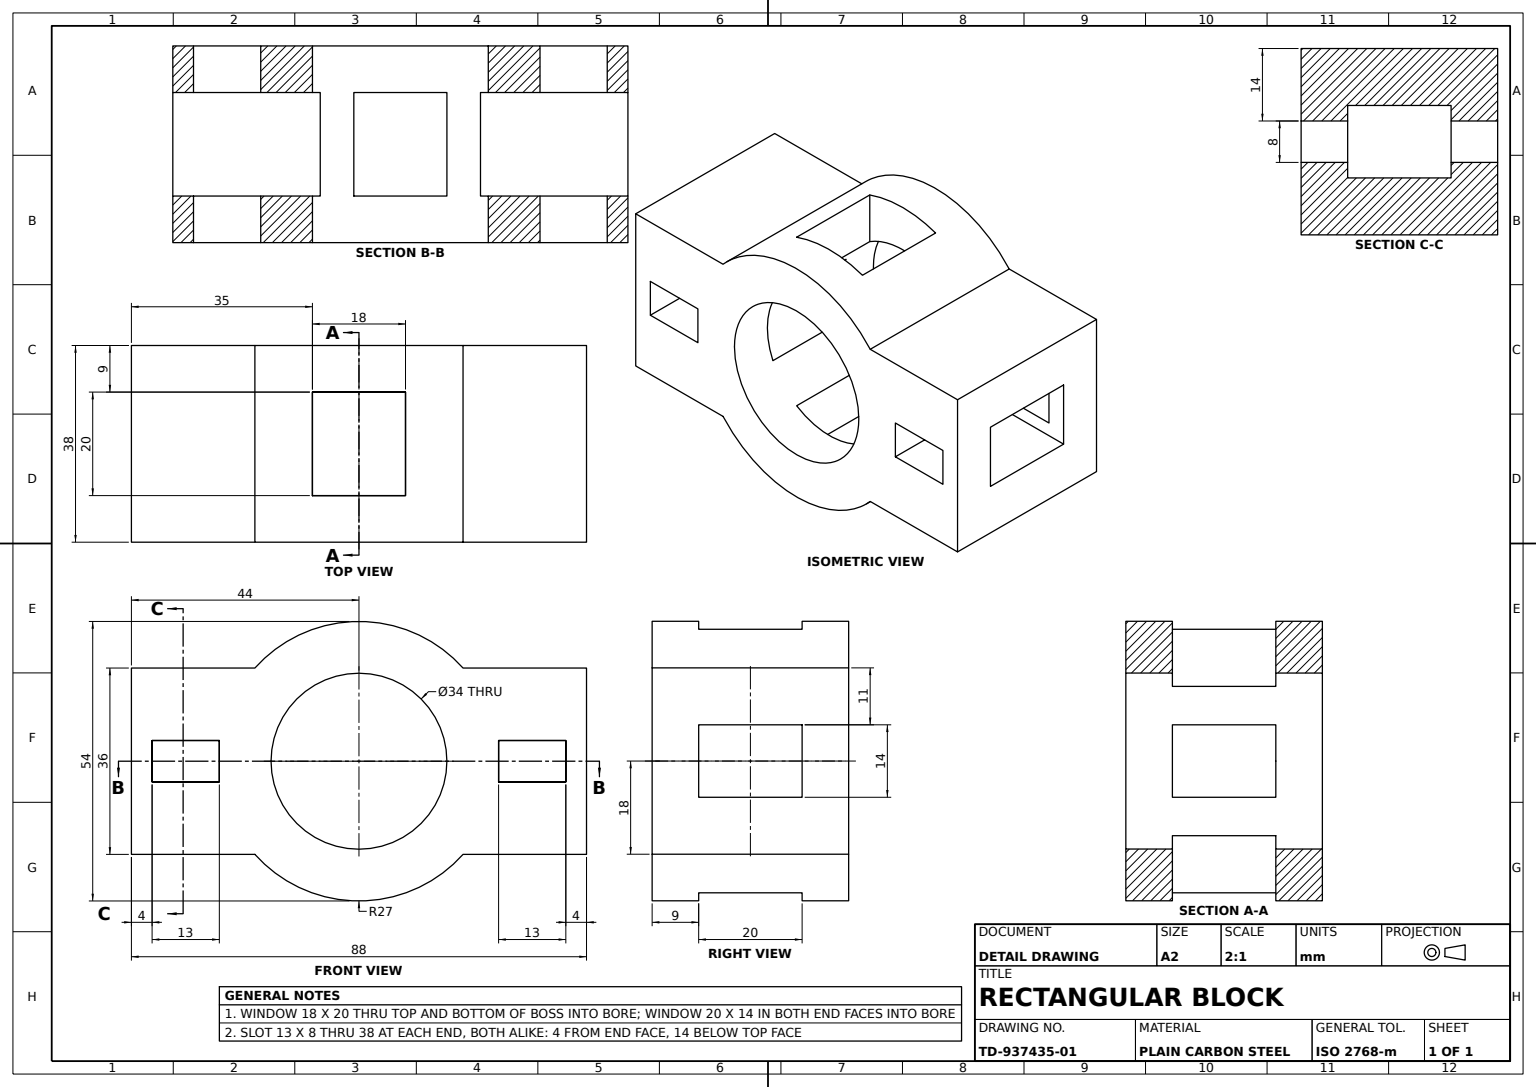
ISO-10303-21;
HEADER;
FILE_DESCRIPTION((''),'2;1');
FILE_NAME('','',(''),(''),'','','');
FILE_SCHEMA(('AUTOMOTIVE_DESIGN'));
ENDSEC;
DATA;
#1=APPLICATION_CONTEXT('');
#2=PRODUCT_CONTEXT('',#1,'mechanical');
#3=PRODUCT('','','',(#2));
#4=PRODUCT_DEFINITION_FORMATION('','',#3);
#5=PRODUCT_DEFINITION_CONTEXT('',#1,'design');
#6=PRODUCT_DEFINITION('','',#4,#5);
#7=PRODUCT_DEFINITION_SHAPE('','',#6);
#8=(LENGTH_UNIT()NAMED_UNIT(*)SI_UNIT(.MILLI.,.METRE.));
#9=(NAMED_UNIT(*)PLANE_ANGLE_UNIT()SI_UNIT($,.RADIAN.));
#10=(NAMED_UNIT(*)SI_UNIT($,.STERADIAN.)SOLID_ANGLE_UNIT());
#11=UNCERTAINTY_MEASURE_WITH_UNIT(LENGTH_MEASURE(1.E-05),#8,'distance_accuracy_value','');
#12=(GEOMETRIC_REPRESENTATION_CONTEXT(3)GLOBAL_UNCERTAINTY_ASSIGNED_CONTEXT((#11))GLOBAL_UNIT_ASSIGNED_CONTEXT((#8,#9,#10))REPRESENTATION_CONTEXT('',''));
#13=CARTESIAN_POINT('',(9.,14.422205,-29.));
#14=VERTEX_POINT('',#13);
#15=CARTESIAN_POINT('',(9.,14.422205,-9.));
#16=VERTEX_POINT('',#15);
#17=CARTESIAN_POINT('',(9.,14.422205,-38.));
#18=DIRECTION('',(0.,0.,1.));
#19=VECTOR('',#18,1000.);
#20=LINE('',#17,#19);
#21=EDGE_CURVE('',#14,#16,#20,.T.);
#22=ORIENTED_EDGE('',*,*,#21,.T.);
#23=CARTESIAN_POINT('',(9.,25.455844,-9.));
#24=VERTEX_POINT('',#23);
#25=CARTESIAN_POINT('',(9.,27.,-9.));
#26=DIRECTION('',(0.,-1.,0.));
#27=VECTOR('',#26,1000.);
#28=LINE('',#25,#27);
#29=EDGE_CURVE('',#24,#16,#28,.T.);
#30=ORIENTED_EDGE('',*,*,#29,.F.);
#31=CARTESIAN_POINT('',(9.,25.455844,-29.));
#32=VERTEX_POINT('',#31);
#33=CARTESIAN_POINT('',(9.,25.455844,-38.));
#34=LINE('',#33,#19);
#35=EDGE_CURVE('',#32,#24,#34,.T.);
#36=ORIENTED_EDGE('',*,*,#35,.F.);
#37=CARTESIAN_POINT('',(9.,27.,-29.));
#38=LINE('',#37,#27);
#39=EDGE_CURVE('',#32,#14,#38,.T.);
#40=ORIENTED_EDGE('',*,*,#39,.T.);
#41=EDGE_LOOP('',(#22,#30,#36,#40));
#42=FACE_OUTER_BOUND('',#41,.T.);
#43=DIRECTION('',(-1.,0.,0.));
#44=AXIS2_PLACEMENT_3D('',#25,#43,#18);
#45=PLANE('',#44);
#46=ADVANCED_FACE('',(#42),#45,.T.);
#47=CARTESIAN_POINT('',(44.,7.,-9.));
#48=VERTEX_POINT('',#47);
#49=CARTESIAN_POINT('',(15.491933,7.,-9.));
#50=VERTEX_POINT('',#49);
#51=VECTOR('',#43,1000.);
#52=LINE('',#47,#51);
#53=EDGE_CURVE('',#48,#50,#52,.T.);
#54=ORIENTED_EDGE('',*,*,#53,.F.);
#55=CARTESIAN_POINT('',(44.,-7.,-9.));
#56=VERTEX_POINT('',#55);
#57=DIRECTION('',(0.,1.,0.));
#58=VECTOR('',#57,1000.);
#59=LINE('',#55,#58);
#60=EDGE_CURVE('',#56,#48,#59,.T.);
#61=ORIENTED_EDGE('',*,*,#60,.F.);
#62=CARTESIAN_POINT('',(15.491933,-7.,-9.));
#63=VERTEX_POINT('',#62);
#64=LINE('',#55,#51);
#65=EDGE_CURVE('',#56,#63,#64,.T.);
#66=ORIENTED_EDGE('',*,*,#65,.T.);
#67=CARTESIAN_POINT('',(17.,0.,-9.));
#68=VERTEX_POINT('',#67);
#69=CARTESIAN_POINT('',(0.,0.,-9.));
#70=DIRECTION('',(0.,0.,-1.));
#71=DIRECTION('',(1.,0.,0.));
#72=AXIS2_PLACEMENT_3D('',#69,#70,#71);
#73=CIRCLE('',#72,17.);
#74=EDGE_CURVE('',#68,#63,#73,.T.);
#75=ORIENTED_EDGE('',*,*,#74,.F.);
#76=EDGE_CURVE('',#50,#68,#73,.T.);
#77=ORIENTED_EDGE('',*,*,#76,.F.);
#78=EDGE_LOOP('',(#54,#61,#66,#75,#77));
#79=FACE_OUTER_BOUND('',#78,.T.);
#80=CARTESIAN_POINT('',(27.,4.,-9.));
#81=VERTEX_POINT('',#80);
#82=CARTESIAN_POINT('',(40.,4.,-9.));
#83=VERTEX_POINT('',#82);
#84=VECTOR('',#71,1000.);
#85=LINE('',#82,#84);
#86=EDGE_CURVE('',#81,#83,#85,.T.);
#87=ORIENTED_EDGE('',*,*,#86,.F.);
#88=CARTESIAN_POINT('',(27.,-4.,-9.));
#89=VERTEX_POINT('',#88);
#90=LINE('',#88,#58);
#91=EDGE_CURVE('',#89,#81,#90,.T.);
#92=ORIENTED_EDGE('',*,*,#91,.F.);
#93=CARTESIAN_POINT('',(40.,-4.,-9.));
#94=VERTEX_POINT('',#93);
#95=LINE('',#93,#51);
#96=EDGE_CURVE('',#94,#89,#95,.T.);
#97=ORIENTED_EDGE('',*,*,#96,.F.);
#98=LINE('',#93,#27);
#99=EDGE_CURVE('',#83,#94,#98,.T.);
#100=ORIENTED_EDGE('',*,*,#99,.F.);
#101=EDGE_LOOP('',(#87,#92,#97,#100));
#102=FACE_BOUND('',#101,.T.);
#103=AXIS2_PLACEMENT_3D('',#55,#18,#71);
#104=PLANE('',#103);
#105=ADVANCED_FACE('',(#79,#102),#104,.F.);
#106=CARTESIAN_POINT('',(-15.491933,-7.,-29.));
#107=VERTEX_POINT('',#106);
#108=CARTESIAN_POINT('',(-15.491933,-7.,-9.));
#109=VERTEX_POINT('',#108);
#110=CARTESIAN_POINT('',(-15.491933,-7.,-38.));
#111=LINE('',#110,#19);
#112=EDGE_CURVE('',#107,#109,#111,.T.);
#113=ORIENTED_EDGE('',*,*,#112,.F.);
#114=CARTESIAN_POINT('',(-44.,-7.,-29.));
#115=VERTEX_POINT('',#114);
#116=CARTESIAN_POINT('',(44.,-7.,-29.));
#117=LINE('',#116,#51);
#118=EDGE_CURVE('',#107,#115,#117,.T.);
#119=ORIENTED_EDGE('',*,*,#118,.T.);
#120=CARTESIAN_POINT('',(-44.,-7.,-9.));
#121=VERTEX_POINT('',#120);
#122=CARTESIAN_POINT('',(-44.,-7.,-38.));
#123=LINE('',#122,#19);
#124=EDGE_CURVE('',#115,#121,#123,.T.);
#125=ORIENTED_EDGE('',*,*,#124,.T.);
#126=EDGE_CURVE('',#109,#121,#64,.T.);
#127=ORIENTED_EDGE('',*,*,#126,.F.);
#128=EDGE_LOOP('',(#113,#119,#125,#127));
#129=FACE_OUTER_BOUND('',#128,.T.);
#130=AXIS2_PLACEMENT_3D('',#116,#26,#70);
#131=PLANE('',#130);
#132=ADVANCED_FACE('',(#129),#131,.F.);
#133=CARTESIAN_POINT('',(15.491933,-7.,-29.));
#134=VERTEX_POINT('',#133);
#135=CARTESIAN_POINT('',(15.491933,-7.,-38.));
#136=VECTOR('',#70,1000.);
#137=LINE('',#135,#136);
#138=EDGE_CURVE('',#63,#134,#137,.T.);
#139=ORIENTED_EDGE('',*,*,#138,.F.);
#140=ORIENTED_EDGE('',*,*,#65,.F.);
#141=VERTEX_POINT('',#116);
#142=LINE('',#116,#19);
#143=EDGE_CURVE('',#141,#56,#142,.T.);
#144=ORIENTED_EDGE('',*,*,#143,.F.);
#145=EDGE_CURVE('',#141,#134,#117,.T.);
#146=ORIENTED_EDGE('',*,*,#145,.T.);
#147=EDGE_LOOP('',(#139,#140,#144,#146));
#148=FACE_OUTER_BOUND('',#147,.T.);
#149=ADVANCED_FACE('',(#148),#131,.F.);
#150=CARTESIAN_POINT('',(20.124612,-18.,-38.));
#151=VERTEX_POINT('',#150);
#152=CARTESIAN_POINT('',(20.124612,-18.,0.));
#153=VERTEX_POINT('',#152);
#154=LINE('',#150,#19);
#155=EDGE_CURVE('',#151,#153,#154,.T.);
#156=ORIENTED_EDGE('',*,*,#155,.F.);
#157=CARTESIAN_POINT('',(44.,-18.,-38.));
#158=VERTEX_POINT('',#157);
#159=LINE('',#150,#84);
#160=EDGE_CURVE('',#151,#158,#159,.T.);
#161=ORIENTED_EDGE('',*,*,#160,.T.);
#162=CARTESIAN_POINT('',(44.,-18.,0.));
#163=VERTEX_POINT('',#162);
#164=LINE('',#157,#19);
#165=EDGE_CURVE('',#158,#163,#164,.T.);
#166=ORIENTED_EDGE('',*,*,#165,.T.);
#167=LINE('',#152,#84);
#168=EDGE_CURVE('',#153,#163,#167,.T.);
#169=ORIENTED_EDGE('',*,*,#168,.F.);
#170=EDGE_LOOP('',(#156,#161,#166,#169));
#171=FACE_OUTER_BOUND('',#170,.T.);
#172=AXIS2_PLACEMENT_3D('',#150,#26,#70);
#173=PLANE('',#172);
#174=ADVANCED_FACE('',(#171),#173,.T.);
#175=CARTESIAN_POINT('',(9.,-14.422205,-9.));
#176=VERTEX_POINT('',#175);
#177=CARTESIAN_POINT('',(9.,-14.422205,-29.));
#178=VERTEX_POINT('',#177);
#179=CARTESIAN_POINT('',(9.,-14.422205,-38.));
#180=LINE('',#179,#136);
#181=EDGE_CURVE('',#176,#178,#180,.T.);
#182=ORIENTED_EDGE('',*,*,#181,.F.);
#183=CARTESIAN_POINT('',(-9.,-14.422205,-9.));
#184=VERTEX_POINT('',#183);
#185=AXIS2_PLACEMENT_3D('',#69,#18,#43);
#186=CIRCLE('',#185,17.);
#187=EDGE_CURVE('',#184,#176,#186,.T.);
#188=ORIENTED_EDGE('',*,*,#187,.F.);
#189=CARTESIAN_POINT('',(-9.,-14.422205,-29.));
#190=VERTEX_POINT('',#189);
#191=CARTESIAN_POINT('',(-9.,-14.422205,-38.));
#192=LINE('',#191,#19);
#193=EDGE_CURVE('',#190,#184,#192,.T.);
#194=ORIENTED_EDGE('',*,*,#193,.F.);
#195=CARTESIAN_POINT('',(0.,0.,-29.));
#196=AXIS2_PLACEMENT_3D('',#195,#70,#71);
#197=CIRCLE('',#196,17.);
#198=EDGE_CURVE('',#178,#190,#197,.T.);
#199=ORIENTED_EDGE('',*,*,#198,.F.);
#200=EDGE_LOOP('',(#182,#188,#194,#199));
#201=FACE_BOUND('',#200,.T.);
#202=CARTESIAN_POINT('',(17.,0.,0.));
#203=VERTEX_POINT('',#202);
#204=CARTESIAN_POINT('',(17.,0.,-38.));
#205=LINE('',#204,#19);
#206=EDGE_CURVE('',#68,#203,#205,.T.);
#207=ORIENTED_EDGE('',*,*,#206,.F.);
#208=ORIENTED_EDGE('',*,*,#74,.T.);
#209=ORIENTED_EDGE('',*,*,#138,.T.);
#210=CARTESIAN_POINT('',(17.,0.,-29.));
#211=VERTEX_POINT('',#210);
#212=AXIS2_PLACEMENT_3D('',#195,#18,#43);
#213=CIRCLE('',#212,17.);
#214=EDGE_CURVE('',#134,#211,#213,.T.);
#215=ORIENTED_EDGE('',*,*,#214,.T.);
#216=VERTEX_POINT('',#204);
#217=EDGE_CURVE('',#216,#211,#205,.T.);
#218=ORIENTED_EDGE('',*,*,#217,.F.);
#219=CARTESIAN_POINT('',(-17.,0.,-38.));
#220=VERTEX_POINT('',#219);
#221=CARTESIAN_POINT('',(0.,0.,-38.));
#222=AXIS2_PLACEMENT_3D('',#221,#18,#71);
#223=CIRCLE('',#222,17.);
#224=EDGE_CURVE('',#220,#216,#223,.T.);
#225=ORIENTED_EDGE('',*,*,#224,.F.);
#226=CARTESIAN_POINT('',(-17.,0.,-29.));
#227=VERTEX_POINT('',#226);
#228=LINE('',#219,#19);
#229=EDGE_CURVE('',#220,#227,#228,.T.);
#230=ORIENTED_EDGE('',*,*,#229,.T.);
#231=EDGE_CURVE('',#227,#107,#213,.T.);
#232=ORIENTED_EDGE('',*,*,#231,.T.);
#233=ORIENTED_EDGE('',*,*,#112,.T.);
#234=CARTESIAN_POINT('',(-17.,0.,-9.));
#235=VERTEX_POINT('',#234);
#236=EDGE_CURVE('',#109,#235,#73,.T.);
#237=ORIENTED_EDGE('',*,*,#236,.T.);
#238=CARTESIAN_POINT('',(-17.,0.,0.));
#239=VERTEX_POINT('',#238);
#240=EDGE_CURVE('',#235,#239,#228,.T.);
#241=ORIENTED_EDGE('',*,*,#240,.T.);
#242=CARTESIAN_POINT('',(0.,0.,0.));
#243=AXIS2_PLACEMENT_3D('',#242,#18,#71);
#244=CIRCLE('',#243,17.);
#245=EDGE_CURVE('',#239,#203,#244,.T.);
#246=ORIENTED_EDGE('',*,*,#245,.T.);
#247=EDGE_LOOP('',(#207,#208,#209,#215,#218,#225,#230,#232,#233,#237,#241,#246));
#248=FACE_OUTER_BOUND('',#247,.T.);
#249=CYLINDRICAL_SURFACE('',#222,17.);
#250=ADVANCED_FACE('',(#201,#248),#249,.F.);
#251=CARTESIAN_POINT('',(-20.124612,18.,0.));
#252=VERTEX_POINT('',#251);
#253=CARTESIAN_POINT('',(-44.,18.,0.));
#254=VERTEX_POINT('',#253);
#255=LINE('',#253,#51);
#256=EDGE_CURVE('',#252,#254,#255,.T.);
#257=ORIENTED_EDGE('',*,*,#256,.F.);
#258=CARTESIAN_POINT('',(-20.124612,18.,-38.));
#259=VERTEX_POINT('',#258);
#260=LINE('',#258,#19);
#261=EDGE_CURVE('',#259,#252,#260,.T.);
#262=ORIENTED_EDGE('',*,*,#261,.F.);
#263=CARTESIAN_POINT('',(-44.,18.,-38.));
#264=VERTEX_POINT('',#263);
#265=LINE('',#263,#51);
#266=EDGE_CURVE('',#259,#264,#265,.T.);
#267=ORIENTED_EDGE('',*,*,#266,.T.);
#268=LINE('',#263,#19);
#269=EDGE_CURVE('',#264,#254,#268,.T.);
#270=ORIENTED_EDGE('',*,*,#269,.T.);
#271=EDGE_LOOP('',(#257,#262,#267,#270));
#272=FACE_OUTER_BOUND('',#271,.T.);
#273=AXIS2_PLACEMENT_3D('',#263,#57,#18);
#274=PLANE('',#273);
#275=ADVANCED_FACE('',(#272),#274,.T.);
#276=CARTESIAN_POINT('',(-44.,7.,-9.));
#277=VERTEX_POINT('',#276);
#278=CARTESIAN_POINT('',(-44.,7.,-29.));
#279=VERTEX_POINT('',#278);
#280=CARTESIAN_POINT('',(-44.,7.,-38.));
#281=LINE('',#280,#136);
#282=EDGE_CURVE('',#277,#279,#281,.T.);
#283=ORIENTED_EDGE('',*,*,#282,.T.);
#284=CARTESIAN_POINT('',(-15.491933,7.,-29.));
#285=VERTEX_POINT('',#284);
#286=CARTESIAN_POINT('',(44.,7.,-29.));
#287=LINE('',#286,#51);
#288=EDGE_CURVE('',#285,#279,#287,.T.);
#289=ORIENTED_EDGE('',*,*,#288,.F.);
#290=CARTESIAN_POINT('',(-15.491933,7.,-9.));
#291=VERTEX_POINT('',#290);
#292=CARTESIAN_POINT('',(-15.491933,7.,-38.));
#293=LINE('',#292,#136);
#294=EDGE_CURVE('',#291,#285,#293,.T.);
#295=ORIENTED_EDGE('',*,*,#294,.F.);
#296=EDGE_CURVE('',#291,#277,#52,.T.);
#297=ORIENTED_EDGE('',*,*,#296,.T.);
#298=EDGE_LOOP('',(#283,#289,#295,#297));
#299=FACE_OUTER_BOUND('',#298,.T.);
#300=AXIS2_PLACEMENT_3D('',#286,#57,#18);
#301=PLANE('',#300);
#302=ADVANCED_FACE('',(#299),#301,.F.);
#303=CARTESIAN_POINT('',(-40.,-4.,0.));
#304=VERTEX_POINT('',#303);
#305=CARTESIAN_POINT('',(-27.,-4.,0.));
#306=VERTEX_POINT('',#305);
#307=LINE('',#303,#84);
#308=EDGE_CURVE('',#304,#306,#307,.T.);
#309=ORIENTED_EDGE('',*,*,#308,.T.);
#310=CARTESIAN_POINT('',(-27.,-4.,-9.));
#311=VERTEX_POINT('',#310);
#312=CARTESIAN_POINT('',(-27.,-4.,-38.));
#313=LINE('',#312,#19);
#314=EDGE_CURVE('',#311,#306,#313,.T.);
#315=ORIENTED_EDGE('',*,*,#314,.F.);
#316=CARTESIAN_POINT('',(-40.,-4.,-9.));
#317=VERTEX_POINT('',#316);
#318=LINE('',#316,#51);
#319=EDGE_CURVE('',#311,#317,#318,.T.);
#320=ORIENTED_EDGE('',*,*,#319,.T.);
#321=CARTESIAN_POINT('',(-40.,-4.,-38.));
#322=LINE('',#321,#19);
#323=EDGE_CURVE('',#317,#304,#322,.T.);
#324=ORIENTED_EDGE('',*,*,#323,.T.);
#325=EDGE_LOOP('',(#309,#315,#320,#324));
#326=FACE_OUTER_BOUND('',#325,.T.);
#327=AXIS2_PLACEMENT_3D('',#321,#26,#70);
#328=PLANE('',#327);
#329=ADVANCED_FACE('',(#326),#328,.F.);
#330=CARTESIAN_POINT('',(-9.,25.455844,-29.));
#331=VERTEX_POINT('',#330);
#332=CARTESIAN_POINT('',(-9.,14.422205,-29.));
#333=VERTEX_POINT('',#332);
#334=CARTESIAN_POINT('',(-9.,27.,-29.));
#335=LINE('',#334,#27);
#336=EDGE_CURVE('',#331,#333,#335,.T.);
#337=ORIENTED_EDGE('',*,*,#336,.T.);
#338=EDGE_CURVE('',#333,#14,#197,.T.);
#339=ORIENTED_EDGE('',*,*,#338,.T.);
#340=ORIENTED_EDGE('',*,*,#39,.F.);
#341=CIRCLE('',#196,27.);
#342=EDGE_CURVE('',#331,#32,#341,.T.);
#343=ORIENTED_EDGE('',*,*,#342,.F.);
#344=EDGE_LOOP('',(#337,#339,#340,#343));
#345=FACE_OUTER_BOUND('',#344,.T.);
#346=AXIS2_PLACEMENT_3D('',#334,#18,#71);
#347=PLANE('',#346);
#348=ADVANCED_FACE('',(#345),#347,.T.);
#349=CARTESIAN_POINT('',(-27.,4.,-9.));
#350=VERTEX_POINT('',#349);
#351=CARTESIAN_POINT('',(-27.,4.,0.));
#352=VERTEX_POINT('',#351);
#353=CARTESIAN_POINT('',(-27.,4.,-38.));
#354=LINE('',#353,#19);
#355=EDGE_CURVE('',#350,#352,#354,.T.);
#356=ORIENTED_EDGE('',*,*,#355,.T.);
#357=CARTESIAN_POINT('',(-40.,4.,0.));
#358=VERTEX_POINT('',#357);
#359=LINE('',#357,#51);
#360=EDGE_CURVE('',#352,#358,#359,.T.);
#361=ORIENTED_EDGE('',*,*,#360,.T.);
#362=CARTESIAN_POINT('',(-40.,4.,-9.));
#363=VERTEX_POINT('',#362);
#364=CARTESIAN_POINT('',(-40.,4.,-38.));
#365=LINE('',#364,#19);
#366=EDGE_CURVE('',#363,#358,#365,.T.);
#367=ORIENTED_EDGE('',*,*,#366,.F.);
#368=LINE('',#362,#84);
#369=EDGE_CURVE('',#363,#350,#368,.T.);
#370=ORIENTED_EDGE('',*,*,#369,.T.);
#371=EDGE_LOOP('',(#356,#361,#367,#370));
#372=FACE_OUTER_BOUND('',#371,.T.);
#373=AXIS2_PLACEMENT_3D('',#364,#57,#18);
#374=PLANE('',#373);
#375=ADVANCED_FACE('',(#372),#374,.F.);
#376=CARTESIAN_POINT('',(40.,4.,0.));
#377=VERTEX_POINT('',#376);
#378=CARTESIAN_POINT('',(27.,4.,0.));
#379=VERTEX_POINT('',#378);
#380=LINE('',#376,#51);
#381=EDGE_CURVE('',#377,#379,#380,.T.);
#382=ORIENTED_EDGE('',*,*,#381,.T.);
#383=CARTESIAN_POINT('',(27.,4.,-38.));
#384=LINE('',#383,#19);
#385=EDGE_CURVE('',#81,#379,#384,.T.);
#386=ORIENTED_EDGE('',*,*,#385,.F.);
#387=ORIENTED_EDGE('',*,*,#86,.T.);
#388=CARTESIAN_POINT('',(40.,4.,-38.));
#389=LINE('',#388,#19);
#390=EDGE_CURVE('',#83,#377,#389,.T.);
#391=ORIENTED_EDGE('',*,*,#390,.T.);
#392=EDGE_LOOP('',(#382,#386,#387,#391));
#393=FACE_OUTER_BOUND('',#392,.T.);
#394=AXIS2_PLACEMENT_3D('',#388,#57,#18);
#395=PLANE('',#394);
#396=ADVANCED_FACE('',(#393),#395,.F.);
#397=VERTEX_POINT('',#312);
#398=VERTEX_POINT('',#353);
#399=LINE('',#312,#58);
#400=EDGE_CURVE('',#397,#398,#399,.T.);
#401=ORIENTED_EDGE('',*,*,#400,.F.);
#402=CARTESIAN_POINT('',(-27.,-4.,-29.));
#403=VERTEX_POINT('',#402);
#404=EDGE_CURVE('',#397,#403,#313,.T.);
#405=ORIENTED_EDGE('',*,*,#404,.T.);
#406=CARTESIAN_POINT('',(-27.,4.,-29.));
#407=VERTEX_POINT('',#406);
#408=LINE('',#402,#58);
#409=EDGE_CURVE('',#403,#407,#408,.T.);
#410=ORIENTED_EDGE('',*,*,#409,.T.);
#411=EDGE_CURVE('',#398,#407,#354,.T.);
#412=ORIENTED_EDGE('',*,*,#411,.F.);
#413=EDGE_LOOP('',(#401,#405,#410,#412));
#414=FACE_OUTER_BOUND('',#413,.T.);
#415=AXIS2_PLACEMENT_3D('',#312,#71,#70);
#416=PLANE('',#415);
#417=ADVANCED_FACE('',(#414),#416,.F.);
#418=ORIENTED_EDGE('',*,*,#198,.T.);
#419=CARTESIAN_POINT('',(-9.,-25.455844,-29.));
#420=VERTEX_POINT('',#419);
#421=EDGE_CURVE('',#190,#420,#335,.T.);
#422=ORIENTED_EDGE('',*,*,#421,.T.);
#423=CARTESIAN_POINT('',(9.,-25.455844,-29.));
#424=VERTEX_POINT('',#423);
#425=EDGE_CURVE('',#424,#420,#341,.T.);
#426=ORIENTED_EDGE('',*,*,#425,.F.);
#427=EDGE_CURVE('',#178,#424,#38,.T.);
#428=ORIENTED_EDGE('',*,*,#427,.F.);
#429=EDGE_LOOP('',(#418,#422,#426,#428));
#430=FACE_OUTER_BOUND('',#429,.T.);
#431=ADVANCED_FACE('',(#430),#347,.T.);
#432=ORIENTED_EDGE('',*,*,#96,.T.);
#433=CARTESIAN_POINT('',(27.,-4.,0.));
#434=VERTEX_POINT('',#433);
#435=CARTESIAN_POINT('',(27.,-4.,-38.));
#436=LINE('',#435,#19);
#437=EDGE_CURVE('',#89,#434,#436,.T.);
#438=ORIENTED_EDGE('',*,*,#437,.T.);
#439=CARTESIAN_POINT('',(40.,-4.,0.));
#440=VERTEX_POINT('',#439);
#441=LINE('',#439,#84);
#442=EDGE_CURVE('',#434,#440,#441,.T.);
#443=ORIENTED_EDGE('',*,*,#442,.T.);
#444=CARTESIAN_POINT('',(40.,-4.,-38.));
#445=LINE('',#444,#19);
#446=EDGE_CURVE('',#94,#440,#445,.T.);
#447=ORIENTED_EDGE('',*,*,#446,.F.);
#448=EDGE_LOOP('',(#432,#438,#443,#447));
#449=FACE_OUTER_BOUND('',#448,.T.);
#450=AXIS2_PLACEMENT_3D('',#444,#26,#70);
#451=PLANE('',#450);
#452=ADVANCED_FACE('',(#449),#451,.F.);
#453=CARTESIAN_POINT('',(-9.,25.455844,-9.));
#454=VERTEX_POINT('',#453);
#455=CARTESIAN_POINT('',(-9.,25.455844,-38.));
#456=LINE('',#455,#136);
#457=EDGE_CURVE('',#454,#331,#456,.T.);
#458=ORIENTED_EDGE('',*,*,#457,.T.);
#459=ORIENTED_EDGE('',*,*,#342,.T.);
#460=ORIENTED_EDGE('',*,*,#35,.T.);
#461=CIRCLE('',#185,27.);
#462=EDGE_CURVE('',#24,#454,#461,.T.);
#463=ORIENTED_EDGE('',*,*,#462,.T.);
#464=EDGE_LOOP('',(#458,#459,#460,#463));
#465=FACE_BOUND('',#464,.T.);
#466=CARTESIAN_POINT('',(20.124612,18.,-38.));
#467=VERTEX_POINT('',#466);
#468=CARTESIAN_POINT('',(20.124612,18.,0.));
#469=VERTEX_POINT('',#468);
#470=LINE('',#466,#19);
#471=EDGE_CURVE('',#467,#469,#470,.T.);
#472=ORIENTED_EDGE('',*,*,#471,.F.);
#473=CIRCLE('',#222,27.);
#474=EDGE_CURVE('',#467,#259,#473,.T.);
#475=ORIENTED_EDGE('',*,*,#474,.T.);
#476=ORIENTED_EDGE('',*,*,#261,.T.);
#477=CIRCLE('',#243,27.);
#478=EDGE_CURVE('',#469,#252,#477,.T.);
#479=ORIENTED_EDGE('',*,*,#478,.F.);
#480=EDGE_LOOP('',(#472,#475,#476,#479));
#481=FACE_OUTER_BOUND('',#480,.T.);
#482=CYLINDRICAL_SURFACE('',#222,27.);
#483=ADVANCED_FACE('',(#465,#481),#482,.T.);
#484=ORIENTED_EDGE('',*,*,#437,.F.);
#485=ORIENTED_EDGE('',*,*,#91,.T.);
#486=ORIENTED_EDGE('',*,*,#385,.T.);
#487=LINE('',#433,#27);
#488=EDGE_CURVE('',#379,#434,#487,.T.);
#489=ORIENTED_EDGE('',*,*,#488,.T.);
#490=EDGE_LOOP('',(#484,#485,#486,#489));
#491=FACE_OUTER_BOUND('',#490,.T.);
#492=AXIS2_PLACEMENT_3D('',#435,#43,#18);
#493=PLANE('',#492);
#494=ADVANCED_FACE('',(#491),#493,.F.);
#495=ORIENTED_EDGE('',*,*,#404,.F.);
#496=VERTEX_POINT('',#321);
#497=LINE('',#321,#84);
#498=EDGE_CURVE('',#496,#397,#497,.T.);
#499=ORIENTED_EDGE('',*,*,#498,.F.);
#500=CARTESIAN_POINT('',(-40.,-4.,-29.));
#501=VERTEX_POINT('',#500);
#502=EDGE_CURVE('',#496,#501,#322,.T.);
#503=ORIENTED_EDGE('',*,*,#502,.T.);
#504=LINE('',#500,#84);
#505=EDGE_CURVE('',#501,#403,#504,.T.);
#506=ORIENTED_EDGE('',*,*,#505,.T.);
#507=EDGE_LOOP('',(#495,#499,#503,#506));
#508=FACE_OUTER_BOUND('',#507,.T.);
#509=ADVANCED_FACE('',(#508),#328,.F.);
#510=VERTEX_POINT('',#383);
#511=CARTESIAN_POINT('',(27.,4.,-29.));
#512=VERTEX_POINT('',#511);
#513=EDGE_CURVE('',#510,#512,#384,.T.);
#514=ORIENTED_EDGE('',*,*,#513,.T.);
#515=CARTESIAN_POINT('',(27.,-4.,-29.));
#516=VERTEX_POINT('',#515);
#517=LINE('',#515,#27);
#518=EDGE_CURVE('',#512,#516,#517,.T.);
#519=ORIENTED_EDGE('',*,*,#518,.T.);
#520=VERTEX_POINT('',#435);
#521=EDGE_CURVE('',#520,#516,#436,.T.);
#522=ORIENTED_EDGE('',*,*,#521,.F.);
#523=LINE('',#435,#27);
#524=EDGE_CURVE('',#510,#520,#523,.T.);
#525=ORIENTED_EDGE('',*,*,#524,.F.);
#526=EDGE_LOOP('',(#514,#519,#522,#525));
#527=FACE_OUTER_BOUND('',#526,.T.);
#528=ADVANCED_FACE('',(#527),#493,.F.);
#529=ORIENTED_EDGE('',*,*,#366,.T.);
#530=LINE('',#303,#27);
#531=EDGE_CURVE('',#358,#304,#530,.T.);
#532=ORIENTED_EDGE('',*,*,#531,.T.);
#533=ORIENTED_EDGE('',*,*,#323,.F.);
#534=LINE('',#316,#58);
#535=EDGE_CURVE('',#317,#363,#534,.T.);
#536=ORIENTED_EDGE('',*,*,#535,.T.);
#537=EDGE_LOOP('',(#529,#532,#533,#536));
#538=FACE_OUTER_BOUND('',#537,.T.);
#539=AXIS2_PLACEMENT_3D('',#321,#43,#18);
#540=PLANE('',#539);
#541=ADVANCED_FACE('',(#538),#540,.F.);
#542=ORIENTED_EDGE('',*,*,#513,.F.);
#543=VERTEX_POINT('',#388);
#544=LINE('',#388,#51);
#545=EDGE_CURVE('',#543,#510,#544,.T.);
#546=ORIENTED_EDGE('',*,*,#545,.F.);
#547=CARTESIAN_POINT('',(40.,4.,-29.));
#548=VERTEX_POINT('',#547);
#549=EDGE_CURVE('',#543,#548,#389,.T.);
#550=ORIENTED_EDGE('',*,*,#549,.T.);
#551=LINE('',#547,#51);
#552=EDGE_CURVE('',#548,#512,#551,.T.);
#553=ORIENTED_EDGE('',*,*,#552,.T.);
#554=EDGE_LOOP('',(#542,#546,#550,#553));
#555=FACE_OUTER_BOUND('',#554,.T.);
#556=ADVANCED_FACE('',(#555),#395,.F.);
#557=ORIENTED_EDGE('',*,*,#336,.F.);
#558=ORIENTED_EDGE('',*,*,#457,.F.);
#559=CARTESIAN_POINT('',(-9.,14.422205,-9.));
#560=VERTEX_POINT('',#559);
#561=CARTESIAN_POINT('',(-9.,27.,-9.));
#562=LINE('',#561,#27);
#563=EDGE_CURVE('',#454,#560,#562,.T.);
#564=ORIENTED_EDGE('',*,*,#563,.T.);
#565=CARTESIAN_POINT('',(-9.,14.422205,-38.));
#566=LINE('',#565,#136);
#567=EDGE_CURVE('',#560,#333,#566,.T.);
#568=ORIENTED_EDGE('',*,*,#567,.T.);
#569=EDGE_LOOP('',(#557,#558,#564,#568));
#570=FACE_OUTER_BOUND('',#569,.T.);
#571=AXIS2_PLACEMENT_3D('',#561,#71,#70);
#572=PLANE('',#571);
#573=ADVANCED_FACE('',(#570),#572,.T.);
#574=ORIENTED_EDGE('',*,*,#502,.F.);
#575=VERTEX_POINT('',#364);
#576=LINE('',#321,#27);
#577=EDGE_CURVE('',#575,#496,#576,.T.);
#578=ORIENTED_EDGE('',*,*,#577,.F.);
#579=CARTESIAN_POINT('',(-40.,4.,-29.));
#580=VERTEX_POINT('',#579);
#581=EDGE_CURVE('',#575,#580,#365,.T.);
#582=ORIENTED_EDGE('',*,*,#581,.T.);
#583=LINE('',#500,#27);
#584=EDGE_CURVE('',#580,#501,#583,.T.);
#585=ORIENTED_EDGE('',*,*,#584,.T.);
#586=EDGE_LOOP('',(#574,#578,#582,#585));
#587=FACE_OUTER_BOUND('',#586,.T.);
#588=ADVANCED_FACE('',(#587),#540,.F.);
#589=LINE('',#305,#58);
#590=EDGE_CURVE('',#306,#352,#589,.T.);
#591=ORIENTED_EDGE('',*,*,#590,.T.);
#592=ORIENTED_EDGE('',*,*,#355,.F.);
#593=LINE('',#310,#27);
#594=EDGE_CURVE('',#350,#311,#593,.T.);
#595=ORIENTED_EDGE('',*,*,#594,.T.);
#596=ORIENTED_EDGE('',*,*,#314,.T.);
#597=EDGE_LOOP('',(#591,#592,#595,#596));
#598=FACE_OUTER_BOUND('',#597,.T.);
#599=ADVANCED_FACE('',(#598),#416,.F.);
#600=CARTESIAN_POINT('',(-9.,-25.455844,-9.));
#601=VERTEX_POINT('',#600);
#602=CARTESIAN_POINT('',(-9.,-25.455844,-38.));
#603=LINE('',#602,#19);
#604=EDGE_CURVE('',#420,#601,#603,.T.);
#605=ORIENTED_EDGE('',*,*,#604,.F.);
#606=ORIENTED_EDGE('',*,*,#421,.F.);
#607=ORIENTED_EDGE('',*,*,#193,.T.);
#608=EDGE_CURVE('',#184,#601,#562,.T.);
#609=ORIENTED_EDGE('',*,*,#608,.T.);
#610=EDGE_LOOP('',(#605,#606,#607,#609));
#611=FACE_OUTER_BOUND('',#610,.T.);
#612=ADVANCED_FACE('',(#611),#572,.T.);
#613=CARTESIAN_POINT('',(-44.,-18.,0.));
#614=VERTEX_POINT('',#613);
#615=LINE('',#613,#27);
#616=EDGE_CURVE('',#254,#614,#615,.T.);
#617=ORIENTED_EDGE('',*,*,#616,.F.);
#618=ORIENTED_EDGE('',*,*,#269,.F.);
#619=CARTESIAN_POINT('',(-44.,-18.,-38.));
#620=VERTEX_POINT('',#619);
#621=LINE('',#619,#27);
#622=EDGE_CURVE('',#264,#620,#621,.T.);
#623=ORIENTED_EDGE('',*,*,#622,.T.);
#624=LINE('',#619,#19);
#625=EDGE_CURVE('',#620,#614,#624,.T.);
#626=ORIENTED_EDGE('',*,*,#625,.T.);
#627=EDGE_LOOP('',(#617,#618,#623,#626));
#628=FACE_OUTER_BOUND('',#627,.T.);
#629=ORIENTED_EDGE('',*,*,#124,.F.);
#630=CARTESIAN_POINT('',(-44.,-18.,-29.));
#631=LINE('',#630,#27);
#632=EDGE_CURVE('',#279,#115,#631,.T.);
#633=ORIENTED_EDGE('',*,*,#632,.F.);
#634=ORIENTED_EDGE('',*,*,#282,.F.);
#635=CARTESIAN_POINT('',(-44.,-18.,-9.));
#636=LINE('',#635,#58);
#637=EDGE_CURVE('',#121,#277,#636,.T.);
#638=ORIENTED_EDGE('',*,*,#637,.F.);
#639=EDGE_LOOP('',(#629,#633,#634,#638));
#640=FACE_BOUND('',#639,.T.);
#641=AXIS2_PLACEMENT_3D('',#619,#43,#18);
#642=PLANE('',#641);
#643=ADVANCED_FACE('',(#628,#640),#642,.T.);
#644=CARTESIAN_POINT('',(9.,-25.455844,-9.));
#645=VERTEX_POINT('',#644);
#646=EDGE_CURVE('',#176,#645,#28,.T.);
#647=ORIENTED_EDGE('',*,*,#646,.T.);
#648=EDGE_CURVE('',#601,#645,#461,.T.);
#649=ORIENTED_EDGE('',*,*,#648,.F.);
#650=ORIENTED_EDGE('',*,*,#608,.F.);
#651=ORIENTED_EDGE('',*,*,#187,.T.);
#652=EDGE_LOOP('',(#647,#649,#650,#651));
#653=FACE_OUTER_BOUND('',#652,.T.);
#654=AXIS2_PLACEMENT_3D('',#561,#70,#43);
#655=PLANE('',#654);
#656=ADVANCED_FACE('',(#653),#655,.T.);
#657=ORIENTED_EDGE('',*,*,#296,.F.);
#658=EDGE_CURVE('',#235,#291,#73,.T.);
#659=ORIENTED_EDGE('',*,*,#658,.F.);
#660=ORIENTED_EDGE('',*,*,#236,.F.);
#661=ORIENTED_EDGE('',*,*,#126,.T.);
#662=ORIENTED_EDGE('',*,*,#637,.T.);
#663=EDGE_LOOP('',(#657,#659,#660,#661,#662));
#664=FACE_OUTER_BOUND('',#663,.T.);
#665=ORIENTED_EDGE('',*,*,#535,.F.);
#666=ORIENTED_EDGE('',*,*,#319,.F.);
#667=ORIENTED_EDGE('',*,*,#594,.F.);
#668=ORIENTED_EDGE('',*,*,#369,.F.);
#669=EDGE_LOOP('',(#665,#666,#667,#668));
#670=FACE_BOUND('',#669,.T.);
#671=ADVANCED_FACE('',(#664,#670),#104,.F.);
#672=CARTESIAN_POINT('',(44.,18.,-38.));
#673=VERTEX_POINT('',#672);
#674=LINE('',#157,#58);
#675=EDGE_CURVE('',#158,#673,#674,.T.);
#676=ORIENTED_EDGE('',*,*,#675,.T.);
#677=CARTESIAN_POINT('',(44.,18.,0.));
#678=VERTEX_POINT('',#677);
#679=LINE('',#672,#19);
#680=EDGE_CURVE('',#673,#678,#679,.T.);
#681=ORIENTED_EDGE('',*,*,#680,.T.);
#682=LINE('',#162,#58);
#683=EDGE_CURVE('',#163,#678,#682,.T.);
#684=ORIENTED_EDGE('',*,*,#683,.F.);
#685=ORIENTED_EDGE('',*,*,#165,.F.);
#686=EDGE_LOOP('',(#676,#681,#684,#685));
#687=FACE_OUTER_BOUND('',#686,.T.);
#688=ORIENTED_EDGE('',*,*,#143,.T.);
#689=ORIENTED_EDGE('',*,*,#60,.T.);
#690=VERTEX_POINT('',#286);
#691=LINE('',#286,#136);
#692=EDGE_CURVE('',#48,#690,#691,.T.);
#693=ORIENTED_EDGE('',*,*,#692,.T.);
#694=LINE('',#116,#27);
#695=EDGE_CURVE('',#690,#141,#694,.T.);
#696=ORIENTED_EDGE('',*,*,#695,.T.);
#697=EDGE_LOOP('',(#688,#689,#693,#696));
#698=FACE_BOUND('',#697,.T.);
#699=AXIS2_PLACEMENT_3D('',#157,#71,#70);
#700=PLANE('',#699);
#701=ADVANCED_FACE('',(#687,#698),#700,.T.);
#702=CARTESIAN_POINT('',(40.,-4.,-29.));
#703=VERTEX_POINT('',#702);
#704=LINE('',#702,#58);
#705=EDGE_CURVE('',#703,#548,#704,.T.);
#706=ORIENTED_EDGE('',*,*,#705,.T.);
#707=ORIENTED_EDGE('',*,*,#549,.F.);
#708=VERTEX_POINT('',#444);
#709=LINE('',#444,#58);
#710=EDGE_CURVE('',#708,#543,#709,.T.);
#711=ORIENTED_EDGE('',*,*,#710,.F.);
#712=EDGE_CURVE('',#708,#703,#445,.T.);
#713=ORIENTED_EDGE('',*,*,#712,.T.);
#714=EDGE_LOOP('',(#706,#707,#711,#713));
#715=FACE_OUTER_BOUND('',#714,.T.);
#716=AXIS2_PLACEMENT_3D('',#444,#71,#70);
#717=PLANE('',#716);
#718=ADVANCED_FACE('',(#715),#717,.F.);
#719=ORIENTED_EDGE('',*,*,#214,.F.);
#720=ORIENTED_EDGE('',*,*,#145,.F.);
#721=ORIENTED_EDGE('',*,*,#695,.F.);
#722=CARTESIAN_POINT('',(15.491933,7.,-29.));
#723=VERTEX_POINT('',#722);
#724=EDGE_CURVE('',#690,#723,#287,.T.);
#725=ORIENTED_EDGE('',*,*,#724,.T.);
#726=EDGE_CURVE('',#211,#723,#213,.T.);
#727=ORIENTED_EDGE('',*,*,#726,.F.);
#728=EDGE_LOOP('',(#719,#720,#721,#725,#727));
#729=FACE_OUTER_BOUND('',#728,.T.);
#730=ORIENTED_EDGE('',*,*,#705,.F.);
#731=LINE('',#702,#84);
#732=EDGE_CURVE('',#516,#703,#731,.T.);
#733=ORIENTED_EDGE('',*,*,#732,.F.);
#734=ORIENTED_EDGE('',*,*,#518,.F.);
#735=ORIENTED_EDGE('',*,*,#552,.F.);
#736=EDGE_LOOP('',(#730,#733,#734,#735));
#737=FACE_BOUND('',#736,.T.);
#738=AXIS2_PLACEMENT_3D('',#116,#70,#43);
#739=PLANE('',#738);
#740=ADVANCED_FACE('',(#729,#737),#739,.F.);
#741=ORIENTED_EDGE('',*,*,#446,.T.);
#742=LINE('',#439,#58);
#743=EDGE_CURVE('',#440,#377,#742,.T.);
#744=ORIENTED_EDGE('',*,*,#743,.T.);
#745=ORIENTED_EDGE('',*,*,#390,.F.);
#746=ORIENTED_EDGE('',*,*,#99,.T.);
#747=EDGE_LOOP('',(#741,#744,#745,#746));
#748=FACE_OUTER_BOUND('',#747,.T.);
#749=ADVANCED_FACE('',(#748),#717,.F.);
#750=ORIENTED_EDGE('',*,*,#21,.F.);
#751=ORIENTED_EDGE('',*,*,#338,.F.);
#752=ORIENTED_EDGE('',*,*,#567,.F.);
#753=EDGE_CURVE('',#16,#560,#186,.T.);
#754=ORIENTED_EDGE('',*,*,#753,.F.);
#755=EDGE_LOOP('',(#750,#751,#752,#754));
#756=FACE_BOUND('',#755,.T.);
#757=ORIENTED_EDGE('',*,*,#206,.T.);
#758=EDGE_CURVE('',#203,#239,#244,.T.);
#759=ORIENTED_EDGE('',*,*,#758,.T.);
#760=ORIENTED_EDGE('',*,*,#240,.F.);
#761=ORIENTED_EDGE('',*,*,#658,.T.);
#762=ORIENTED_EDGE('',*,*,#294,.T.);
#763=EDGE_CURVE('',#285,#227,#213,.T.);
#764=ORIENTED_EDGE('',*,*,#763,.T.);
#765=ORIENTED_EDGE('',*,*,#229,.F.);
#766=EDGE_CURVE('',#216,#220,#223,.T.);
#767=ORIENTED_EDGE('',*,*,#766,.F.);
#768=ORIENTED_EDGE('',*,*,#217,.T.);
#769=ORIENTED_EDGE('',*,*,#726,.T.);
#770=CARTESIAN_POINT('',(15.491933,7.,-38.));
#771=LINE('',#770,#19);
#772=EDGE_CURVE('',#723,#50,#771,.T.);
#773=ORIENTED_EDGE('',*,*,#772,.T.);
#774=ORIENTED_EDGE('',*,*,#76,.T.);
#775=EDGE_LOOP('',(#757,#759,#760,#761,#762,#764,#765,#767,#768,#769,#773,#774));
#776=FACE_OUTER_BOUND('',#775,.T.);
#777=ADVANCED_FACE('',(#756,#776),#249,.F.);
#778=ORIENTED_EDGE('',*,*,#505,.F.);
#779=ORIENTED_EDGE('',*,*,#584,.F.);
#780=LINE('',#579,#51);
#781=EDGE_CURVE('',#407,#580,#780,.T.);
#782=ORIENTED_EDGE('',*,*,#781,.F.);
#783=ORIENTED_EDGE('',*,*,#409,.F.);
#784=EDGE_LOOP('',(#778,#779,#782,#783));
#785=FACE_BOUND('',#784,.T.);
#786=ORIENTED_EDGE('',*,*,#231,.F.);
#787=ORIENTED_EDGE('',*,*,#763,.F.);
#788=ORIENTED_EDGE('',*,*,#288,.T.);
#789=ORIENTED_EDGE('',*,*,#632,.T.);
#790=ORIENTED_EDGE('',*,*,#118,.F.);
#791=EDGE_LOOP('',(#786,#787,#788,#789,#790));
#792=FACE_OUTER_BOUND('',#791,.T.);
#793=ADVANCED_FACE('',(#785,#792),#739,.F.);
#794=ORIENTED_EDGE('',*,*,#646,.F.);
#795=ORIENTED_EDGE('',*,*,#181,.T.);
#796=ORIENTED_EDGE('',*,*,#427,.T.);
#797=CARTESIAN_POINT('',(9.,-25.455844,-38.));
#798=LINE('',#797,#136);
#799=EDGE_CURVE('',#645,#424,#798,.T.);
#800=ORIENTED_EDGE('',*,*,#799,.F.);
#801=EDGE_LOOP('',(#794,#795,#796,#800));
#802=FACE_OUTER_BOUND('',#801,.T.);
#803=ADVANCED_FACE('',(#802),#45,.T.);
#804=LINE('',#444,#84);
#805=EDGE_CURVE('',#520,#708,#804,.T.);
#806=ORIENTED_EDGE('',*,*,#805,.F.);
#807=ORIENTED_EDGE('',*,*,#521,.T.);
#808=ORIENTED_EDGE('',*,*,#732,.T.);
#809=ORIENTED_EDGE('',*,*,#712,.F.);
#810=EDGE_LOOP('',(#806,#807,#808,#809));
#811=FACE_OUTER_BOUND('',#810,.T.);
#812=ADVANCED_FACE('',(#811),#451,.F.);
#813=ORIENTED_EDGE('',*,*,#29,.T.);
#814=ORIENTED_EDGE('',*,*,#753,.T.);
#815=ORIENTED_EDGE('',*,*,#563,.F.);
#816=ORIENTED_EDGE('',*,*,#462,.F.);
#817=EDGE_LOOP('',(#813,#814,#815,#816));
#818=FACE_OUTER_BOUND('',#817,.T.);
#819=ADVANCED_FACE('',(#818),#655,.T.);
#820=CARTESIAN_POINT('',(-20.124612,-18.,-38.));
#821=VERTEX_POINT('',#820);
#822=LINE('',#619,#84);
#823=EDGE_CURVE('',#620,#821,#822,.T.);
#824=ORIENTED_EDGE('',*,*,#823,.T.);
#825=CARTESIAN_POINT('',(-20.124612,-18.,0.));
#826=VERTEX_POINT('',#825);
#827=LINE('',#820,#19);
#828=EDGE_CURVE('',#821,#826,#827,.T.);
#829=ORIENTED_EDGE('',*,*,#828,.T.);
#830=LINE('',#613,#84);
#831=EDGE_CURVE('',#614,#826,#830,.T.);
#832=ORIENTED_EDGE('',*,*,#831,.F.);
#833=ORIENTED_EDGE('',*,*,#625,.F.);
#834=EDGE_LOOP('',(#824,#829,#832,#833));
#835=FACE_OUTER_BOUND('',#834,.T.);
#836=AXIS2_PLACEMENT_3D('',#619,#26,#70);
#837=PLANE('',#836);
#838=ADVANCED_FACE('',(#835),#837,.T.);
#839=EDGE_CURVE('',#821,#151,#473,.T.);
#840=ORIENTED_EDGE('',*,*,#839,.T.);
#841=ORIENTED_EDGE('',*,*,#155,.T.);
#842=EDGE_CURVE('',#826,#153,#477,.T.);
#843=ORIENTED_EDGE('',*,*,#842,.F.);
#844=ORIENTED_EDGE('',*,*,#828,.F.);
#845=EDGE_LOOP('',(#840,#841,#843,#844));
#846=FACE_OUTER_BOUND('',#845,.T.);
#847=ORIENTED_EDGE('',*,*,#604,.T.);
#848=ORIENTED_EDGE('',*,*,#648,.T.);
#849=ORIENTED_EDGE('',*,*,#799,.T.);
#850=ORIENTED_EDGE('',*,*,#425,.T.);
#851=EDGE_LOOP('',(#847,#848,#849,#850));
#852=FACE_BOUND('',#851,.T.);
#853=ADVANCED_FACE('',(#846,#852),#482,.T.);
#854=LINE('',#466,#51);
#855=EDGE_CURVE('',#673,#467,#854,.T.);
#856=ORIENTED_EDGE('',*,*,#855,.T.);
#857=ORIENTED_EDGE('',*,*,#471,.T.);
#858=LINE('',#468,#51);
#859=EDGE_CURVE('',#678,#469,#858,.T.);
#860=ORIENTED_EDGE('',*,*,#859,.F.);
#861=ORIENTED_EDGE('',*,*,#680,.F.);
#862=EDGE_LOOP('',(#856,#857,#860,#861));
#863=FACE_OUTER_BOUND('',#862,.T.);
#864=AXIS2_PLACEMENT_3D('',#466,#57,#18);
#865=PLANE('',#864);
#866=ADVANCED_FACE('',(#863),#865,.T.);
#867=ORIENTED_EDGE('',*,*,#805,.T.);
#868=ORIENTED_EDGE('',*,*,#710,.T.);
#869=ORIENTED_EDGE('',*,*,#545,.T.);
#870=ORIENTED_EDGE('',*,*,#524,.T.);
#871=EDGE_LOOP('',(#867,#868,#869,#870));
#872=FACE_BOUND('',#871,.T.);
#873=LINE('',#364,#51);
#874=EDGE_CURVE('',#398,#575,#873,.T.);
#875=ORIENTED_EDGE('',*,*,#874,.T.);
#876=ORIENTED_EDGE('',*,*,#577,.T.);
#877=ORIENTED_EDGE('',*,*,#498,.T.);
#878=ORIENTED_EDGE('',*,*,#400,.T.);
#879=EDGE_LOOP('',(#875,#876,#877,#878));
#880=FACE_BOUND('',#879,.T.);
#881=ORIENTED_EDGE('',*,*,#224,.T.);
#882=ORIENTED_EDGE('',*,*,#766,.T.);
#883=EDGE_LOOP('',(#881,#882));
#884=FACE_BOUND('',#883,.T.);
#885=ORIENTED_EDGE('',*,*,#622,.F.);
#886=ORIENTED_EDGE('',*,*,#266,.F.);
#887=ORIENTED_EDGE('',*,*,#474,.F.);
#888=ORIENTED_EDGE('',*,*,#855,.F.);
#889=ORIENTED_EDGE('',*,*,#675,.F.);
#890=ORIENTED_EDGE('',*,*,#160,.F.);
#891=ORIENTED_EDGE('',*,*,#839,.F.);
#892=ORIENTED_EDGE('',*,*,#823,.F.);
#893=EDGE_LOOP('',(#885,#886,#887,#888,#889,#890,#891,#892));
#894=FACE_OUTER_BOUND('',#893,.T.);
#895=PLANE('',#222);
#896=ADVANCED_FACE('',(#872,#880,#884,#894),#895,.F.);
#897=ORIENTED_EDGE('',*,*,#411,.T.);
#898=ORIENTED_EDGE('',*,*,#781,.T.);
#899=ORIENTED_EDGE('',*,*,#581,.F.);
#900=ORIENTED_EDGE('',*,*,#874,.F.);
#901=EDGE_LOOP('',(#897,#898,#899,#900));
#902=FACE_OUTER_BOUND('',#901,.T.);
#903=ADVANCED_FACE('',(#902),#374,.F.);
#904=ORIENTED_EDGE('',*,*,#245,.F.);
#905=ORIENTED_EDGE('',*,*,#758,.F.);
#906=EDGE_LOOP('',(#904,#905));
#907=FACE_BOUND('',#906,.T.);
#908=ORIENTED_EDGE('',*,*,#859,.T.);
#909=ORIENTED_EDGE('',*,*,#478,.T.);
#910=ORIENTED_EDGE('',*,*,#256,.T.);
#911=ORIENTED_EDGE('',*,*,#616,.T.);
#912=ORIENTED_EDGE('',*,*,#831,.T.);
#913=ORIENTED_EDGE('',*,*,#842,.T.);
#914=ORIENTED_EDGE('',*,*,#168,.T.);
#915=ORIENTED_EDGE('',*,*,#683,.T.);
#916=EDGE_LOOP('',(#908,#909,#910,#911,#912,#913,#914,#915));
#917=FACE_OUTER_BOUND('',#916,.T.);
#918=ORIENTED_EDGE('',*,*,#381,.F.);
#919=ORIENTED_EDGE('',*,*,#743,.F.);
#920=ORIENTED_EDGE('',*,*,#442,.F.);
#921=ORIENTED_EDGE('',*,*,#488,.F.);
#922=EDGE_LOOP('',(#918,#919,#920,#921));
#923=FACE_BOUND('',#922,.T.);
#924=ORIENTED_EDGE('',*,*,#360,.F.);
#925=ORIENTED_EDGE('',*,*,#590,.F.);
#926=ORIENTED_EDGE('',*,*,#308,.F.);
#927=ORIENTED_EDGE('',*,*,#531,.F.);
#928=EDGE_LOOP('',(#924,#925,#926,#927));
#929=FACE_BOUND('',#928,.T.);
#930=PLANE('',#243);
#931=ADVANCED_FACE('',(#907,#917,#923,#929),#930,.T.);
#932=ORIENTED_EDGE('',*,*,#772,.F.);
#933=ORIENTED_EDGE('',*,*,#724,.F.);
#934=ORIENTED_EDGE('',*,*,#692,.F.);
#935=ORIENTED_EDGE('',*,*,#53,.T.);
#936=EDGE_LOOP('',(#932,#933,#934,#935));
#937=FACE_OUTER_BOUND('',#936,.T.);
#938=ADVANCED_FACE('',(#937),#301,.F.);
#939=CLOSED_SHELL('',(#46,#105,#132,#149,#174,#250,#275,#302,#329,#348,#375,#396,#417,#431,#452,#483,#494,#509,#528,#541,#556,#573,#588,#599,#612,#643,#656,#671,#701,#718,#740,#749,#777,#793,#803,#812,#819,#838,#853,#866,#896,#903,#931,#938));
#940=MANIFOLD_SOLID_BREP('',#939);
#941=ADVANCED_BREP_SHAPE_REPRESENTATION('',(#940),#12);
#942=SHAPE_DEFINITION_REPRESENTATION(#7,#941);
ENDSEC;
END-ISO-10303-21;
